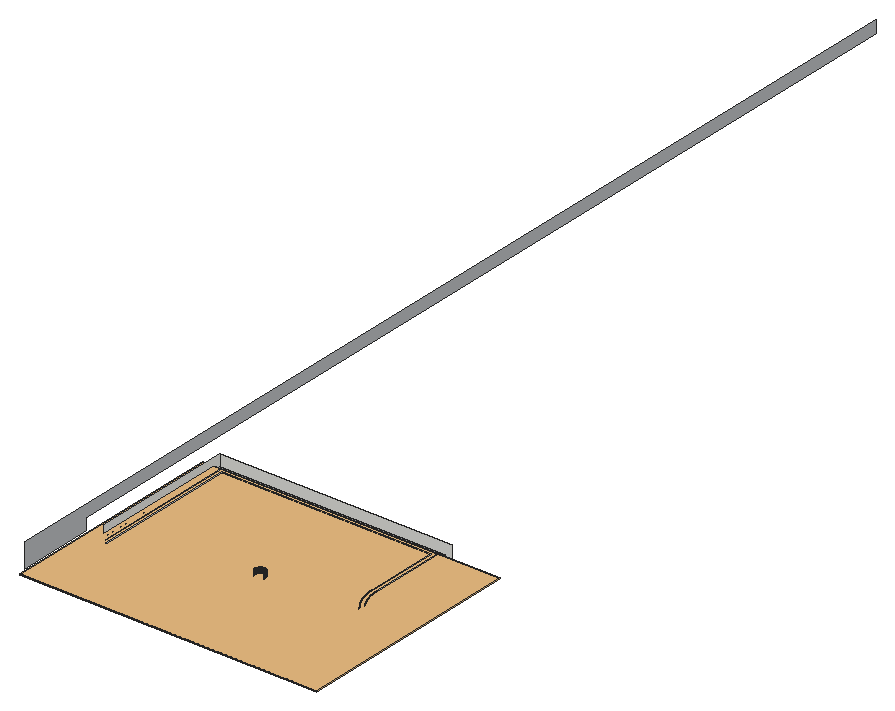
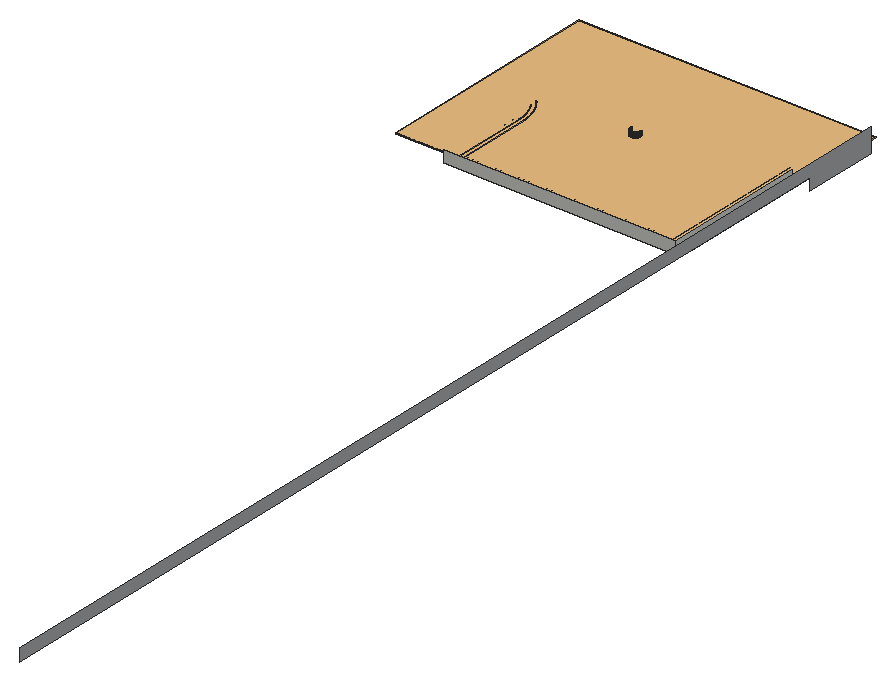
# SketchUp Ruby script. Lengths in inches.
U = 1.inch
M = Sketchup.active_model
def pt(a) = Geom::Point3d.new(a.map { |v| v * U })
def face(e, loops, mat)
  f = e.add_face(loops[0].map { |a| pt(a) })
  loops[1..].each { |l| e.add_face(l.map { |a| pt(a) }).erase! }
  f.material = f.back_material = mat if mat
  f
end
# faces: each face lists its corners as indices into pts; further lists are holes
def faces(e, pts, list, mat = nil) = list.each { |f| face(e, (f[0].is_a?(Array) ? f : [f]).map { |l| l.map { |i| pts[i] } }, mat) }
# xy, xz, yz: faces in a plane at the given z, y or x. An outline is a flat list of corners, or four numbers for a rectangle; further outlines are holes
def ring(l) = l.size == 4 ? [[l[0], l[1]], [l[2], l[1]], [l[2], l[3]], [l[0], l[3]]] : l.each_slice(2).to_a
def flat(e, list, mat, &to3) = list.each { |f| face(e, (f[0].is_a?(Array) ? f : [f]).map { |l| ring(l).map { |u, v| to3.(u, v) } }, mat) }
def xy(e, z, list, mat = nil) = flat(e, list, mat) { |x, y| [x, y, z] }
def xz(e, y, list, mat = nil) = flat(e, list, mat) { |x, z| [x, y, z] }
def yz(e, x, list, mat = nil) = flat(e, list, mat) { |y, z| [x, y, z] }
def lines(e, pts, list) = list.each { |a, b| e.add_line(pt(pts[a]), pt(pts[b])) }
# prism: a flat outline (further loops are holes) pulled along v
def prism(e, loops, v, mat = nil)
  f = face(e, loops, mat); d = Geom::Vector3d.new(v.map { |x| x * U })
  f.pushpull(f.normal.samedirection?(d) ? d.length : -d.length)
end
def box(e, o, s, mat = nil) = prism(e, [[o, [o[0] + s[0], o[1], o[2]], [o[0] + s[0], o[1] + s[1], o[2]], [o[0], o[1] + s[1], o[2]]]], [0, 0, s[2]], mat)
def at(x, y, z, deg = 0) = Geom::Transformation.translation(pt([x, y, z])) * Geom::Transformation.rotation(ORIGIN, Z_AXIS, deg.degrees)
def axes(o, x, y, z) = Geom::Transformation.new([*x, 0, *y, 0, *z, 0, *pt(o).to_a, 1])
def part(name) = M.definitions.add(name)
# library, detail: a bought-in or finely detailed component or shape, given as its bounding box
def library(name, o, s) = part(name).tap { |d| box(d.entities, o, s) }
def detail(e, o, s) = box(e.add_group.entities, o, s)
def put(e, d, t, mat = nil) = e.add_instance(d, t).tap { |i| i.material = mat if mat }
def group(e, t, mat = nil) = e.add_group.tap { |g| g.transformation = t; g.material = mat if mat }.entities
root = M.entities
M.materials.add("1427 AP 686 ARMOUR-N").color = [184, 186, 189]
M.materials.add("False Ceiling Light").color = [251, 213, 131]
c1 = library("Group\#32",[0,0,0],[148,114.08,0.5])
xz(root,193.5,[[86.84,242,86.92,245],[86.92,242,87,245],[87,242,87.08,245],[87.08,242,87.16,245]])
xz(root,246,[[24,242,128,242.5]])
xz(root,248,[[22,242,130,242.5]])
xz(root,250,[[20,240,132,242]],"1427 AP 686 ARMOUR-N")
xz(root,252,[[18,240,134,246]])
yz(root,9,[[141.92,240,141.92,252,672,252,672,246,180,246,180,240]],"1427 AP 686 ARMOUR-N")
yz(root,18,[[180,240,252,246]])
yz(root,20,[[178,240,250,242]],"1427 AP 686 ARMOUR-N")
yz(root,22,[[176,242,248,242.5]])
yz(root,24,[[174,242,246,242.5]])
yz(root,84.5,[[190.84,242,190.92,245],[190.92,242,191,245],[191,242,191.08,245],[191.08,242,191.16,245]])
yz(root,89.5,[[190.84,242,190.92,245],[190.92,242,191,245],[191,242,191.08,245],[191.08,242,191.16,245]])
yz(root,128,[[209.71,242,209.95,242.5],[209.95,242,246,242.5]])
yz(root,130,[[209.73,242,209.96,242.5],[209.96,242,248,242.5]])
yz(root,130.01,[[209.2,242,209.47,242.5]])
yz(root,132,[[209.76,240,209.97,242],[209.97,240,250,242]],"1427 AP 686 ARMOUR-N")
yz(root,132.01,[[209.28,240,209.52,242]],"1427 AP 686 ARMOUR-N")
p = [[133.66,202.01,240],[133.76,201.79,240],[133.76,201.79,242],[133.66,202.01,242],[133.57,202.23,240],[133.57,202.23,242],
  [133.48,202.46,240],[133.48,202.46,242],[133.39,202.68,240],[133.39,202.68,242],[133.3,202.91,240],[133.3,202.91,242],
  [133.22,203.13,240],[133.22,203.13,242],[133.13,203.36,240],[133.13,203.36,242],[133.05,203.59,240],[133.05,203.59,242],
  [132.98,203.82,240],[132.98,203.82,242],[132.91,204.05,240],[132.91,204.05,242],[132.83,204.28,240],[132.83,204.28,242],
  [132.77,204.51,240],[132.77,204.51,242],[132.7,204.75,240],[132.7,204.75,242],[132.64,204.98,240],[132.64,204.98,242],
  [132.58,205.21,240],[132.58,205.21,242],[132.52,205.45,240],[132.52,205.45,242],[132.47,205.68,240],[132.47,205.68,242],
  [132.42,205.92,240],[132.42,205.92,242],[132.37,206.16,240],[132.37,206.16,242],[132.33,206.39,240],[132.33,206.39,242],
  [132.29,206.63,240],[132.29,206.63,242],[132.25,206.87,240],[132.25,206.87,242],[132.21,207.11,240],[132.21,207.11,242],
  [132.18,207.35,240],[132.18,207.35,242],[132.15,207.59,240],[132.15,207.59,242],[132.12,207.83,240],[132.12,207.83,242],
  [132.09,208.07,240],[132.09,208.07,242],[132.07,208.31,240],[132.07,208.31,242],[132.05,208.55,240],[132.05,208.55,242],
  [132.04,208.79,240],[132.04,208.79,242],[132.02,209.03,240],[132.02,209.03,242],[132.01,209.28,240],[132.01,209.28,242],
  [132,209.76,240],[132.01,209.52,240],[132.01,209.52,242],[132,209.76,242],[84.54,190.53,242],[84.53,190.61,242],
  [84.53,190.61,245],[84.54,190.53,245],[84.56,190.45,242],[84.56,190.45,245],[89.46,190.53,242],[89.44,190.45,242],
  [89.44,190.45,245],[89.46,190.53,245],[89.47,190.61,242],[89.47,190.61,245],[84.52,190.6875,242],[84.52,190.6875,245],
  [89.48,190.6875,242],[89.48,190.6875,245],[84.51,190.76,242],[84.51,190.76,245],[89.49,190.76,242],[89.49,190.76,245],
  [84.5,190.84,242],[84.5,190.84,245],[89.5,190.84,242],[89.5,190.84,245],[84.5,191.16,242],[84.51,191.24,242],
  [84.51,191.24,245],[84.5,191.16,245],[84.52,191.3125,242],[84.52,191.3125,245],[89.48,191.3125,242],[89.49,191.24,242],
  [89.49,191.24,245],[89.48,191.3125,245],[89.5,191.16,242],[89.5,191.16,245],[84.53,191.39,242],[84.53,191.39,245],
  [89.47,191.39,242],[89.47,191.39,245],[84.54,191.47,242],[84.54,191.47,245],[89.46,191.47,242],[89.46,191.47,245],
  [84.56,191.55,242],[84.56,191.55,245],[84.58,191.62,242],[84.58,191.62,245],[89.42,191.62,242],[89.44,191.55,242],
  [89.44,191.55,245],[89.42,191.62,245],[84.6,191.7,242],[84.6,191.7,245],[89.4,191.7,242],[89.4,191.7,245],
  [84.62,191.77,242],[84.62,191.77,245],[89.38,191.77,242],[89.38,191.77,245],[84.65,191.85,242],[84.65,191.85,245],
  [84.68,191.92,242],[84.68,191.92,245],[89.32,191.92,242],[89.35,191.85,242],[89.35,191.85,245],[89.32,191.92,245],
  [84.71,191.99,242],[84.71,191.99,245],[89.29,191.99,242],[89.29,191.99,245],[84.74,192.0625,242],[84.74,192.0625,245],
  [89.26,192.0625,242],[89.26,192.0625,245],[84.77,192.13,242],[84.77,192.13,245],[84.81,192.2,242],[84.81,192.2,245],
  [89.19,192.2,242],[89.23,192.13,242],[89.23,192.13,245],[89.19,192.2,245],[84.85,192.27,242],[84.85,192.27,245],
  [89.15,192.27,242],[89.15,192.27,245],[84.89,192.34,242],[84.89,192.34,245],[84.93,192.41,242],[84.93,192.41,245],
  [89.07,192.41,242],[89.11,192.34,242],[89.11,192.34,245],[89.07,192.41,245],[84.98,192.47,242],[84.98,192.47,245],
  [89.02,192.47,242],[89.02,192.47,245],[85.02,192.53,242],[85.02,192.53,245],[85.07,192.59,242],[85.07,192.59,245],
  [88.93,192.59,242],[88.98,192.53,242],[88.98,192.53,245],[88.93,192.59,245],[85.125,192.65,242],[85.125,192.65,245],
  [88.875,192.65,242],[88.875,192.65,245],[85.18,192.71,242],[85.18,192.71,245],[85.23,192.77,242],[85.23,192.77,245],
  [88.77,192.77,242],[88.82,192.71,242],[88.82,192.71,245],[88.77,192.77,245],[85.29,192.82,242],[85.29,192.82,245],
  [85.35,192.875,242],[85.35,192.875,245],[88.65,192.875,242],[88.71,192.82,242],[88.71,192.82,245],[88.65,192.875,245],
  [85.41,192.93,242],[85.41,192.93,245],[85.47,192.98,242],[85.47,192.98,245],[88.53,192.98,242],[88.59,192.93,242],
  [88.59,192.93,245],[88.53,192.98,245],[85.53,193.02,242],[85.53,193.02,245],[85.59,193.07,242],[85.59,193.07,245],
  [88.41,193.07,242],[88.47,193.02,242],[88.47,193.02,245],[88.41,193.07,245],[85.66,193.11,242],[85.66,193.11,245],
  [85.73,193.15,242],[85.73,193.15,245],[88.27,193.15,242],[88.34,193.11,242],[88.34,193.11,245],[88.27,193.15,245],
  [85.8,193.19,242],[85.8,193.19,245],[85.87,193.23,242],[85.87,193.23,245],[85.9375,193.26,242],[85.9375,193.26,245],
  [88.0625,193.26,242],[88.13,193.23,242],[88.13,193.23,245],[88.0625,193.26,245],[88.2,193.19,242],[88.2,193.19,245],
  [86.01,193.29,242],[86.01,193.29,245],[86.08,193.32,242],[86.08,193.32,245],[86.15,193.35,242],[86.15,193.35,245],
  [87.85,193.35,242],[87.92,193.32,242],[87.92,193.32,245],[87.85,193.35,245],[87.99,193.29,242],[87.99,193.29,245],
  [86.23,193.38,242],[86.23,193.38,245],[86.3,193.4,242],[86.3,193.4,245],[86.38,193.42,242],[86.38,193.42,245],
  [86.45,193.44,242],[86.45,193.44,245],[86.53,193.46,242],[86.53,193.46,245],[87.47,193.46,242],[87.55,193.44,242],
  [87.55,193.44,245],[87.47,193.46,245],[87.62,193.42,242],[87.62,193.42,245],[87.7,193.4,242],[87.7,193.4,245],
  [87.77,193.38,242],[87.77,193.38,245],[86.61,193.47,242],[86.61,193.47,245],[86.6875,193.48,242],[86.6875,193.48,245],
  [86.76,193.49,242],[86.76,193.49,245],[86.84,193.5,242],[86.84,193.5,245],[87.16,193.5,242],[87.24,193.49,242],
  [87.24,193.49,245],[87.16,193.5,245],[87.3125,193.48,242],[87.3125,193.48,245],[87.39,193.47,242],[87.39,193.47,245],
  [133.84,194.3,242],[133.66,194.52,242],[133.66,194.52,242.5],[133.84,194.3,242.5],[133.47,194.75,242],[133.47,194.75,242.5],
  [133.29,194.97,242],[133.29,194.97,242.5],[133.11,195.2,242],[133.11,195.2,242.5],[132.93,195.43,242],[132.93,195.43,242.5],
  [132.76,195.66,242],[132.76,195.66,242.5],[132.58,195.89,242],[132.58,195.89,242.5],[132.41,196.13,242],[132.41,196.13,242.5],
  [132.25,196.37,242],[132.25,196.37,242.5],[132.08,196.61,242],[132.08,196.61,242.5],[131.92,196.85,242],[131.92,196.85,242.5],
  [131.77,197.09,242],[131.77,197.09,242.5],[131.61,197.34,242],[131.61,197.34,242.5],[131.46,197.58,242],[131.46,197.58,242.5],
  [131.3125,197.83,242],[131.3125,197.83,242.5],[133.6,197.94,242],[133.74,197.72,242],[133.74,197.72,242.5],[133.6,197.94,242.5],
  [131.17,198.08,242],[131.17,198.08,242.5],[133.45,198.17,242],[133.45,198.17,242.5],[131.02,198.34,242],[131.02,198.34,242.5],
  [133.3125,198.39,242],[133.3125,198.39,242.5],[130.89,198.59,242],[130.89,198.59,242.5],[133.17,198.62,242],[133.17,198.62,242.5],
  [130.75,198.85,242],[130.75,198.85,242.5],[133.04,198.85,242],[133.04,198.85,242.5],[130.62,199.1,242],[130.62,199.1,242.5],
  [132.9,199.08,242],[132.9,199.08,242.5],[130.49,199.36,242],[130.49,199.36,242.5],[132.77,199.31,242],[132.77,199.31,242.5],
  [132.64,199.54,242],[132.64,199.54,242.5],[130.36,199.625,242],[130.36,199.625,242.5],[132.52,199.78,242],[132.52,199.78,242.5],
  [130.23,199.89,242],[130.23,199.89,242.5],[132.4,200.01,242],[132.4,200.01,242.5],[130.11,200.15,242],[130.11,200.15,242.5],
  [132.28,200.25,242],[132.28,200.25,242.5],[130,200.42,242],[130,200.42,242.5],[132.16,200.49,242],[132.16,200.49,242.5],
  [129.88,200.68,242],[129.88,200.68,242.5],[132.05,200.73,242],[132.05,200.73,242.5],[129.77,200.95,242],[129.77,200.95,242.5],
  [131.9375,200.97,242],[131.9375,200.97,242.5],[129.66,201.22,242],[129.66,201.22,242.5],[131.83,201.21,242],[131.83,201.21,242.5],
  [129.56,201.49,242],[129.56,201.49,242.5],[131.73,201.46,242],[131.73,201.46,242.5],[129.46,201.76,242],[129.46,201.76,242.5],
  [131.625,201.7,242],[131.625,201.7,242.5],[131.53,201.95,242],[131.53,201.95,242.5],[129.36,202.03,242],[129.36,202.03,242.5],
  [129.27,202.31,242],[129.27,202.31,242.5],[131.43,202.2,242],[131.43,202.2,242.5],[131.34,202.45,242],[131.34,202.45,242.5],
  [129.17,202.58,242],[129.17,202.58,242.5],[131.25,202.7,242],[131.25,202.7,242.5],[129.09,202.86,242],[129.09,202.86,242.5],
  [131.16,202.95,242],[131.16,202.95,242.5],[129,203.14,242],[129,203.14,242.5],[131.08,203.2,242],[131.08,203.2,242.5],
  [128.92,203.42,242],[128.92,203.42,242.5],[131,203.45,242],[131,203.45,242.5],[128.84,203.69,242],[128.84,203.69,242.5],
  [130.92,203.71,242],[130.92,203.71,242.5],[128.77,203.98,242],[128.77,203.98,242.5],[130.84,203.96,242],[130.84,203.96,242.5],
  [128.7,204.26,242],[128.7,204.26,242.5],[130.77,204.22,242],[130.77,204.22,242.5],[130.7,204.48,242],[130.7,204.48,242.5],
  [128.63,204.54,242],[128.63,204.54,242.5],[128.57,204.82,242],[128.57,204.82,242.5],[130.64,204.73,242],[130.64,204.73,242.5],
  [130.58,204.99,242],[130.58,204.99,242.5],[128.5,205.1,242],[128.5,205.1,242.5],[130.52,205.25,242],[130.52,205.25,242.5],
  [128.45,205.39,242],[128.45,205.39,242.5],[130.46,205.51,242],[130.46,205.51,242.5],[128.39,205.67,242],[128.39,205.67,242.5],
  [130.41,205.77,242],[130.41,205.77,242.5],[128.34,205.96,242],[128.34,205.96,242.5],[130.36,206.03,242],[130.36,206.03,242.5],
  [128.3,206.25,242],[128.3,206.25,242.5],[130.3125,206.3,242],[130.3125,206.3,242.5],[128.25,206.53,242],[128.25,206.53,242.5],
  [130.27,206.56,242],[130.27,206.56,242.5],[128.21,206.82,242],[128.21,206.82,242.5],[130.23,206.82,242],[130.23,206.82,242.5],
  [128.17,207.11,242],[128.17,207.11,242.5],[130.19,207.08,242],[130.19,207.08,242.5],[128.14,207.4,242],[128.14,207.4,242.5],
  [130.16,207.35,242],[130.16,207.35,242.5],[130.13,207.61,242],[130.13,207.61,242.5],[128.11,207.68,242],[128.11,207.68,242.5],
  [130.1,207.875,242],[130.1,207.875,242.5],[128.09,207.97,242],[128.09,207.97,242.5],[130.08,208.14,242],[130.08,208.14,242.5],
  [128.0625,208.26,242],[128.0625,208.26,242.5],[130.06,208.41,242],[130.06,208.41,242.5],[128.04,208.55,242],[128.04,208.55,242.5],
  [130.04,208.67,242],[130.04,208.67,242.5],[128.03,208.84,242],[128.03,208.84,242.5],[130.03,208.9375,242],[130.03,208.9375,242.5],
  [128.02,209.13,242],[128.02,209.13,242.5],[130.01,209.2,242],[130.01,209.2,242.5],[128.01,209.42,242],[128.01,209.42,242.5],
  [128,209.71,242],[128,209.71,242.5],[130,209.73,242],[130.01,209.47,242],[130.01,209.47,242.5],[130,209.73,242.5]]
faces(root,p,[[0,1,2,3],[4,0,3,5],[6,4,5,7],[8,6,7,9],[10,8,9,11],[12,10,11,13],[14,12,13,15],[16,14,15,17],
  [18,16,17,19],[20,18,19,21],[22,20,21,23],[24,22,23,25],[26,24,25,27],[28,26,27,29],[30,28,29,31],[32,30,31,33],
  [34,32,33,35],[36,34,35,37],[38,36,37,39],[40,38,39,41],[42,40,41,43],[44,42,43,45],[46,44,45,47],[48,46,47,49],
  [50,48,49,51],[52,50,51,53],[54,52,53,55],[56,54,55,57],[58,56,57,59],[60,58,59,61],[62,60,61,63],[64,62,63,65],
  [66,67,68,69]],"1427 AP 686 ARMOUR-N")
faces(root,p,[[70,71,72,73],[74,70,73,75],[76,77,78,79],[80,76,79,81],[71,82,83,72],[84,80,81,85],[82,86,87,83],[88,84,85,89],
  [86,90,91,87],[92,88,89,93],[94,95,96,97],[95,98,99,96],[100,101,102,103],[101,104,105,102],[98,106,107,99],[108,100,103,109],
  [106,110,111,107],[112,108,109,113],[110,114,115,111],[114,116,117,115],[118,119,120,121],[119,112,113,120],[116,122,123,117],[124,118,121,125],
  [122,126,127,123],[128,124,125,129],[126,130,131,127],[130,132,133,131],[134,135,136,137],[135,128,129,136],[132,138,139,133],[140,134,137,141],
  [138,142,143,139],[144,140,141,145],[142,146,147,143],[146,148,149,147],[150,151,152,153],[151,144,145,152],[148,154,155,149],[156,150,153,157],
  [154,158,159,155],[158,160,161,159],[162,163,164,165],[163,156,157,164],[160,166,167,161],[168,162,165,169],[166,170,171,167],[170,172,173,171],
  [174,175,176,177],[175,168,169,176],[172,178,179,173],[180,174,177,181],[178,182,183,179],[182,184,185,183],[186,187,188,189],[187,180,181,188],
  [184,190,191,185],[190,192,193,191],[194,195,196,197],[195,186,189,196],[192,198,199,193],[198,200,201,199],[202,203,204,205],[203,194,197,204],
  [200,206,207,201],[206,208,209,207],[210,211,212,213],[211,202,205,212],[208,214,215,209],[214,216,217,215],[218,219,220,221],[219,210,213,220],
  [216,222,223,217],[222,224,225,223],[224,226,227,225],[228,229,230,231],[229,232,233,230],[232,218,221,233],[226,234,235,227],[234,236,237,235],
  [236,238,239,237],[240,241,242,243],[241,244,245,242],[244,228,231,245],[238,246,247,239],[246,248,249,247],[248,250,251,249],[250,252,253,251],
  [252,254,255,253],[256,257,258,259],[257,260,261,258],[260,262,263,261],[262,264,265,263],[264,240,243,265],[254,266,267,255],[266,268,269,267],
  [268,270,271,269],[270,272,273,271],[274,275,276,277],[275,278,279,276],[278,280,281,279],[280,256,259,281],[282,283,284,285],[283,286,287,284],
  [286,288,289,287],[288,290,291,289],[290,292,293,291],[292,294,295,293],[294,296,297,295],[296,298,299,297],[298,300,301,299],[300,302,303,301],
  [302,304,305,303],[304,306,307,305],[306,308,309,307],[308,310,311,309],[310,312,313,311],[314,315,316,317],[312,318,319,313],[320,314,317,321],
  [318,322,323,319],[324,320,321,325],[322,326,327,323],[328,324,325,329],[326,330,331,327],[332,328,329,333],[330,334,335,331],[336,332,333,337],
  [334,338,339,335],[340,336,337,341],[342,340,341,343],[338,344,345,339],[346,342,343,347],[344,348,349,345],[350,346,347,351],[348,352,353,349],
  [354,350,351,355],[352,356,357,353],[358,354,355,359],[356,360,361,357],[362,358,359,363],[360,364,365,361],[366,362,363,367],[364,368,369,365],
  [370,366,367,371],[368,372,373,369],[374,370,371,375],[372,376,377,373],[378,374,375,379],[380,378,379,381],[376,382,383,377],[382,384,385,383],
  [386,380,381,387],[388,386,387,389],[384,390,391,385],[392,388,389,393],[390,394,395,391],[396,392,393,397],[394,398,399,395],[400,396,397,401],
  [398,402,403,399],[404,400,401,405],[402,406,407,403],[408,404,405,409],[406,410,411,407],[412,408,409,413],[410,414,415,411],[416,412,413,417],
  [418,416,417,419],[414,420,421,415],[420,422,423,421],[424,418,419,425],[426,424,425,427],[422,428,429,423],[430,426,427,431],[428,432,433,429],
  [434,430,431,435],[432,436,437,433],[438,434,435,439],[436,440,441,437],[442,438,439,443],[440,444,445,441],[446,442,443,447],[444,448,449,445],
  [450,446,447,451],[448,452,453,449],[454,450,451,455],[452,456,457,453],[458,454,455,459],[456,460,461,457],[462,458,459,463],[464,462,463,465],
  [460,466,467,461],[468,464,465,469],[466,470,471,467],[472,468,469,473],[470,474,475,471],[476,472,473,477],[474,478,479,475],[480,476,477,481],
  [478,482,483,479],[484,480,481,485],[482,486,487,483],[488,484,485,489],[486,490,491,487],[490,492,493,491],[494,495,496,497]])
put(root,c1,at(13,133.92,242),"False Ceiling Light")
